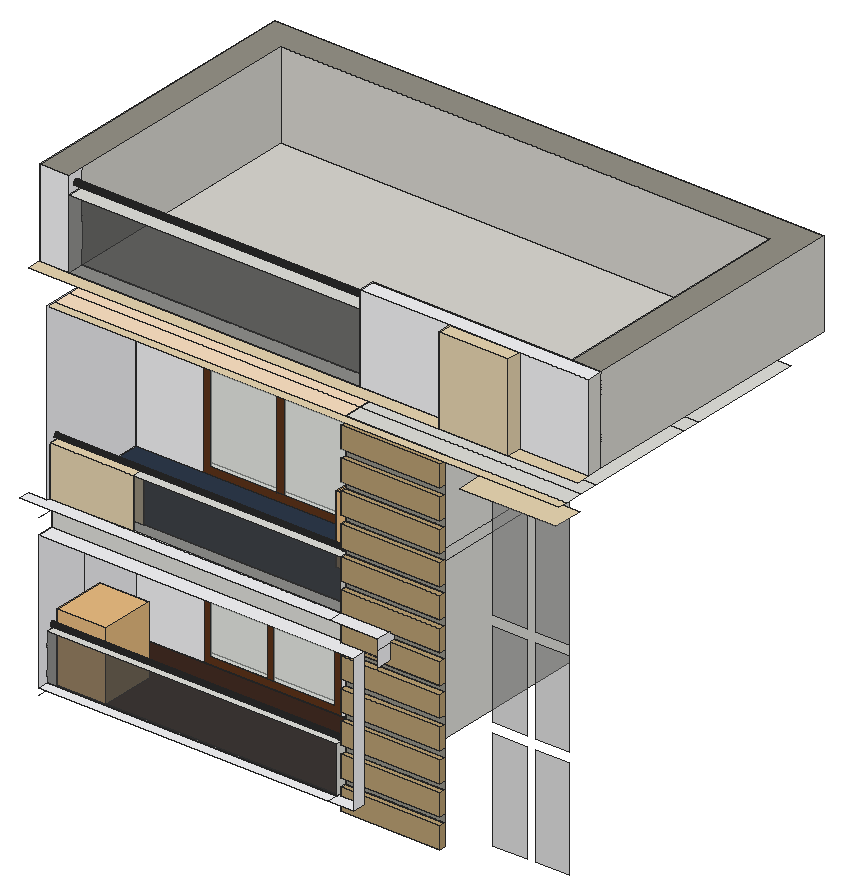
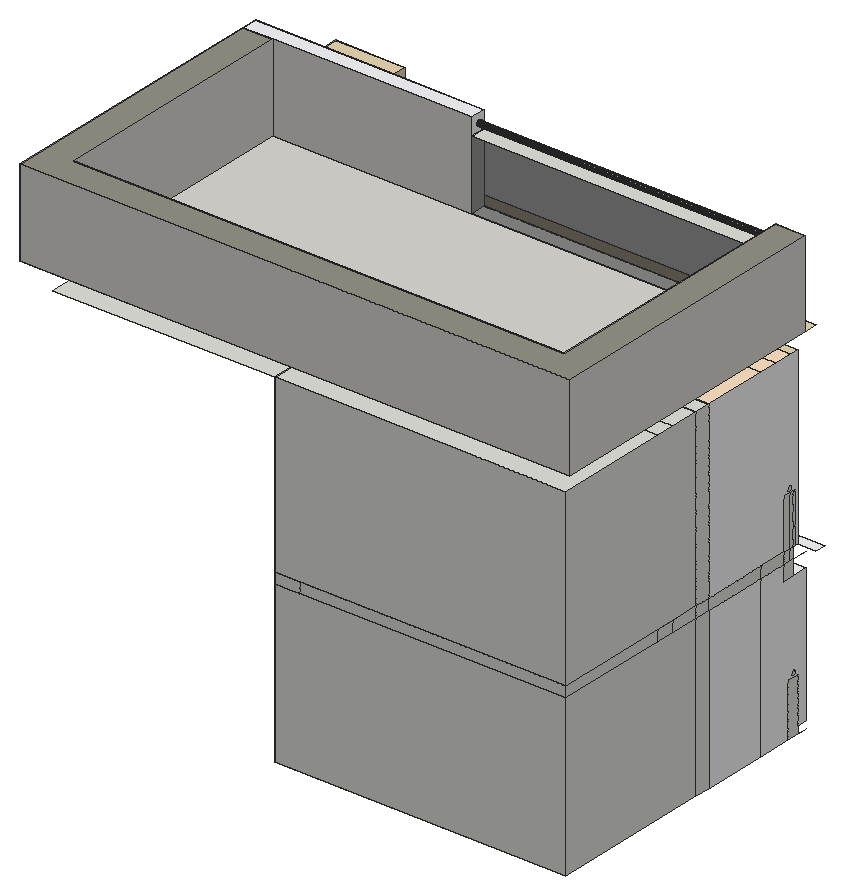
# SketchUp Ruby script. Lengths in inches.
U = 1.inch
M = Sketchup.active_model
def pt(a) = Geom::Point3d.new(a.map { |v| v * U })
def face(e, loops, mat)
  f = e.add_face(loops[0].map { |a| pt(a) })
  loops[1..].each { |l| e.add_face(l.map { |a| pt(a) }).erase! }
  f.material = f.back_material = mat if mat
  f
end
# faces: each face lists its corners as indices into pts; further lists are holes
def faces(e, pts, list, mat = nil) = list.each { |f| face(e, (f[0].is_a?(Array) ? f : [f]).map { |l| l.map { |i| pts[i] } }, mat) }
# xy, xz, yz: faces in a plane at the given z, y or x. An outline is a flat list of corners, or four numbers for a rectangle; further outlines are holes
def ring(l) = l.size == 4 ? [[l[0], l[1]], [l[2], l[1]], [l[2], l[3]], [l[0], l[3]]] : l.each_slice(2).to_a
def flat(e, list, mat, &to3) = list.each { |f| face(e, (f[0].is_a?(Array) ? f : [f]).map { |l| ring(l).map { |u, v| to3.(u, v) } }, mat) }
def xy(e, z, list, mat = nil) = flat(e, list, mat) { |x, y| [x, y, z] }
def xz(e, y, list, mat = nil) = flat(e, list, mat) { |x, z| [x, y, z] }
def yz(e, x, list, mat = nil) = flat(e, list, mat) { |y, z| [x, y, z] }
def lines(e, pts, list) = list.each { |a, b| e.add_line(pt(pts[a]), pt(pts[b])) }
# prism: a flat outline (further loops are holes) pulled along v
def prism(e, loops, v, mat = nil)
  f = face(e, loops, mat); d = Geom::Vector3d.new(v.map { |x| x * U })
  f.pushpull(f.normal.samedirection?(d) ? d.length : -d.length)
end
def box(e, o, s, mat = nil) = prism(e, [[o, [o[0] + s[0], o[1], o[2]], [o[0] + s[0], o[1] + s[1], o[2]], [o[0], o[1] + s[1], o[2]]]], [0, 0, s[2]], mat)
def at(x, y, z, deg = 0) = Geom::Transformation.translation(pt([x, y, z])) * Geom::Transformation.rotation(ORIGIN, Z_AXIS, deg.degrees)
def axes(o, x, y, z) = Geom::Transformation.new([*x, 0, *y, 0, *z, 0, *pt(o).to_a, 1])
def part(name) = M.definitions.add(name)
# library, detail: a bought-in or finely detailed component or shape, given as its bounding box
def library(name, o, s) = part(name).tap { |d| box(d.entities, o, s) }
def detail(e, o, s) = box(e.add_group.entities, o, s)
def put(e, d, t, mat = nil) = e.add_instance(d, t).tap { |i| i.material = mat if mat }
def group(e, t, mat = nil) = e.add_group.tap { |g| g.transformation = t; g.material = mat if mat }.entities
root = M.entities
M.materials.add("[0012_Bisque]").color = [255, 228, 196]
M.materials.add("[Blinds Vertical Pattern]").color = [247, 247, 249]
M.materials.add("[Formica Graystone]").color = [149, 146, 135]
M.materials.add("[Leather Blue]").color = [45, 57, 74]
M.materials.add("[Quartz Light Brown]").color = [234, 216, 179]
M.materials.add("[Suede Brown]").color = [61, 41, 32]
M.materials.add("[Terrazzo Tile Light]").color = [219, 217, 210]
M.materials.add("[Translucent Glass Gray]1").color = [68, 68, 68]
M.materials["[Translucent Glass Gray]1"].alpha = 0.5
M.materials.add("[Translucent Glass Gray]2").color = [128, 128, 128]
M.materials["[Translucent Glass Gray]2"].alpha = 0.5
M.materials.add("[Translucent Glass Safety]1").color = [237, 244, 239]
M.materials["[Translucent Glass Safety]1"].alpha = 0.5
M.materials.add("[Wood Cherry Original]").color = [94, 53, 26]
M.materials.add("[Wood Floor Light]").color = [186, 160, 115]
c1 = library("chau cay",[-24.34,-109.24,0],[56.46,62.58,79.69])
xy(root,479.875,[[484.74,326.3,600.81,332.93]],"[Wood Floor Light]")
xy(root,488.6875,[[144.51,321.91,483.06,335.74],[144.51,452.16,484.74,470.45],[144.51,470.45,484.74,660.02]])
xy(root,488.6875,[[144.51,335.74,483.06,335.74,483.06,341.61,484.74,341.61,484.74,452.16,144.51,452.16]],"[Suede Brown]")
xy(root,496.8125,[[144.51,309.6,483.06,321.91],[483.06,309.6,513.0625,309.6,513.0625,324.41,484.74,324.41,484.74,341.61,483.06,341.61]],"[Blinds Vertical Pattern]")
xy(root,504.8125,[[484.74,326.3,600.81,332.93]],"[Wood Floor Light]")
xy(root,514.3125,[[484.74,326.3,600.81,332.93]],"[Wood Floor Light]")
xy(root,539.25,[[484.74,326.3,600.81,332.93]],"[Wood Floor Light]")
xy(root,548.75,[[484.74,326.3,600.81,332.93]],"[Wood Floor Light]")
xy(root,551,[[144.51,321.91,483.06,335.74]])
xy(root,573.6875,[[484.74,326.3,600.81,332.93]],"[Wood Floor Light]")
xy(root,583.1875,[[484.74,326.3,600.81,332.93]],"[Wood Floor Light]")
xy(root,608.125,[[484.74,326.3,600.81,332.93]],"[Wood Floor Light]")
xy(root,617.625,[[484.74,326.3,600.81,332.93]],"[Wood Floor Light]")
xy(root,642.5625,[[484.74,326.3,600.81,332.93]],"[Wood Floor Light]")
xy(root,652.0625,[[484.74,326.3,600.81,332.93]],"[Wood Floor Light]")
xy(root,656.64,[[144.51,309.6,144.51,328.63,541.38,328.63,541.38,324.41,513.0625,324.41,513.0625,309.6]],"[Blinds Vertical Pattern]")
xy(root,674.6875,[[484.74,326.3,541.38,328.63],[144.51,452.16,484.74,470.45],[144.51,470.45,484.74,660.02]])
xy(root,674.6875,[[144.51,328.63,484.74,452.16]],"[0012_Bisque]")
xy(root,677,[[484.74,326.3,541.38,332.93]])
xy(root,677,[[541.38,326.3,600.81,332.93]],"[Wood Floor Light]")
xy(root,686.5,[[484.74,326.3,541.38,332.93]])
xy(root,686.5,[[541.38,326.3,600.81,332.93]],"[Wood Floor Light]")
xy(root,687.5,[[144.51,326.3,484.74,341.61],[144.51,452.16,484.74,470.45],[144.51,470.45,484.74,660.02]])
xy(root,687.5,[[123.03,309.6,484.74,309.6,484.74,326.3,144.51,326.3,144.51,321.91,123.03,321.91],[484.74,309.6,541.38,326.3]],"[Blinds Vertical Pattern]")
xy(root,687.5,[[144.51,341.61,484.74,452.16]],"[Leather Blue]")
xy(root,711.4375,[[484.74,326.3,600.81,332.93]],"[Wood Floor Light]")
xy(root,720.9375,[[484.74,326.3,600.81,332.93]],"[Wood Floor Light]")
xy(root,745.875,[[242.19,326.3,484.74,341.61]])
xy(root,745.875,[[144.51,326.3,242.19,341.61]],"[Quartz Light Brown]")
xy(root,745.875,[[484.74,326.3,600.81,332.93]],"[Wood Floor Light]")
xy(root,755.375,[[484.74,326.3,600.81,332.93]],"[Wood Floor Light]")
xy(root,780.3125,[[484.74,326.3,600.81,332.93]],"[Wood Floor Light]")
xy(root,789.8125,[[484.74,326.3,600.81,332.93]],"[Wood Floor Light]")
xy(root,814.75,[[484.74,326.3,600.81,332.93]],"[Wood Floor Light]")
xy(root,824.25,[[484.74,326.3,600.81,332.93]],"[Wood Floor Light]")
xy(root,849.1875,[[484.74,326.3,600.81,332.93]],"[Wood Floor Light]")
xy(root,858.6875,[[484.74,326.3,600.81,332.93]],"[Wood Floor Light]")
xy(root,861.54,[[618.4,332.93,730.9,367.24]],"[Quartz Light Brown]")
xy(root,883.625,[[484.74,326.3,600.81,332.93]],"[Wood Floor Light]")
xy(root,890.6875,[[484.74,332.93,743.35,353.85],[484.74,353.85,743.35,375.33],[484.74,375.33,743.35,504.41],[144.51,452.16,484.74,470.45],[144.51,470.45,484.74,504.41],
  [144.51,504.41,484.74,525.85],[484.74,504.41,743.35,525.85],[144.51,525.85,484.74,660.02],[484.74,525.85,743.35,660.02]])
xy(root,890.6875,[[144.51,332.93,484.74,353.85],[144.51,353.85,484.74,375.33],[144.51,375.33,484.74,452.16]],"[0012_Bisque]")
xy(root,890.6875,[[144.51,321.91,743.35,332.93]],"[Quartz Light Brown]")
xy(root,923.6875,[[603.0625,321.91,683.95,338.07],[123.03,338.07,123.03,681.5,764.83,681.5,764.83,356.55,730.2,356.55,730.2,646.87,157.66,646.87,157.66,338.07],[157.66,338.07,497.79,356.55],[497.79,338.07,764.83,356.55]])
xy(root,923.6875,[[123.03,321.91,603.0625,338.07],[683.95,321.91,764.83,338.07]],"[Quartz Light Brown]")
xy(root,923.6875,[[157.66,356.55,730.2,646.87]],"[Terrazzo Tile Light]")
xy(root,1005.0625,[[157.66,338.07,497.79,356.55]])
xy(root,1024.8125,[[497.79,338.07,764.83,356.55]],"[Blinds Vertical Pattern]")
xy(root,1024.8125,[[123.03,338.07,157.66,338.07,157.66,646.87,730.2,646.87,730.2,356.55,764.83,356.55,764.83,681.5,123.03,681.5]],"[Formica Graystone]")
xy(root,1024.8125,[[603.0625,321.91,683.95,338.07]],"[Quartz Light Brown]")
xz(root,321.91,[[144.51,488.6875,483.06,496.8125]])
xz(root,321.91,[[603.0625,923.6875,683.95,1024.8125]],"[Quartz Light Brown]")
xz(root,321.91,[[144.51,496.8125,483.06,551]],"[Translucent Glass Gray]1")
xz(root,326.3,[[484.74,674.6875,541.38,677],[484.74,686.5,541.38,687.5]])
xz(root,326.3,[[144.51,687.5,242.19,745.875]],"[Quartz Light Brown]")
xz(root,326.3,[[242.19,687.5,484.74,745.875]],"[Translucent Glass Gray]1")
xz(root,326.3,[[484.74,479.875,600.81,504.8125],[484.74,514.3125,600.81,539.25],[484.74,548.75,600.81,573.6875],[484.74,583.1875,600.81,608.125],[484.74,617.625,600.81,642.5625],
  [484.74,652.0625,600.81,652.0625,600.81,677,541.38,677,541.38,674.6875,484.74,674.6875],[541.38,686.5,600.81,686.5,600.81,711.4375,484.74,711.4375,484.74,687.5,541.38,687.5],[484.74,720.9375,600.81,745.875],[484.74,755.375,600.81,780.3125],[484.74,789.8125,600.81,814.75],
  [484.74,824.25,600.81,849.1875],[484.74,858.6875,600.81,883.625]],"[Wood Floor Light]")
xz(root,328.63,[[144.51,656.64,541.38,674.6875]])
xz(root,332.93,[[484.74,479.875,600.81,504.8125],[484.74,514.3125,600.81,539.25],[484.74,548.75,600.81,573.6875],[484.74,583.1875,600.81,608.125],[484.74,617.625,600.81,642.5625],
  [484.74,652.0625,600.81,677],[484.74,677,541.38,686.5],[484.74,686.5,600.81,711.4375],[484.74,720.9375,600.81,745.875],[484.74,755.375,600.81,780.3125],
  [484.74,789.8125,600.81,814.75],[484.74,824.25,600.81,849.1875],[484.74,858.6875,600.81,883.625]])
xz(root,332.93,[[484.74,504.8125,600.81,514.3125],[484.74,539.25,600.81,548.75],[484.74,573.6875,600.81,583.1875],[484.74,608.125,600.81,617.625],[484.74,642.5625,600.81,652.0625],
  [541.38,677,600.81,686.5],[484.74,711.4375,600.81,720.9375],[484.74,745.875,600.81,755.375],[484.74,780.3125,600.81,789.8125],[484.74,814.75,600.81,824.25],
  [484.74,849.1875,600.81,858.6875],[484.74,883.625,600.81,890.6875]],"[Formica Graystone]")
xz(root,335.74,[[144.51,488.6875,483.06,551]],"[Translucent Glass Gray]1")
xz(root,338.07,[[603.0625,923.6875,683.95,1024.8125]])
xz(root,338.07,[[123.03,923.6875,157.66,1024.8125],[497.79,923.6875,603.0625,1024.8125],[683.95,923.6875,764.83,1024.8125]],"[Blinds Vertical Pattern]")
xz(root,338.07,[[157.66,923.6875,497.79,1005.0625]],"[Translucent Glass Gray]1")
xz(root,341.61,[[483.06,488.6875,484.74,496.8125]])
xz(root,341.61,[[144.51,687.5,242.19,745.875]],"[Quartz Light Brown]")
xz(root,341.61,[[242.19,687.5,484.74,745.875]],"[Translucent Glass Gray]1")
xz(root,356.55,[[730.2,923.6875,764.83,1024.8125]])
xz(root,356.55,[[497.79,923.6875,730.2,1024.8125]],"[Terrazzo Tile Light]")
xz(root,356.55,[[157.66,923.6875,497.79,1005.0625]],"[Translucent Glass Gray]1")
xz(root,367.24,[[630.125,475.62,670.08,594.34],[679.79,475.62,719.18,594.34],[630.125,604.84,670.08,706.4],[679.79,604.84,719.18,706.4],[630.125,716.91,670.08,849.82],
  [679.79,716.91,719.18,849.82]],"[Translucent Glass Gray]2")
xz(root,452.16,[[144.51,488.6875,223.62,488.6875,223.62,650.375,385.3,650.375,385.3,488.6875,484.74,488.6875,484.74,674.6875,144.51,674.6875],[144.51,687.5,222.91,687.5,222.91,869.9375,405.34,869.9375,405.34,687.5,484.74,687.5,484.74,890.6875,144.51,890.6875]],"[Blinds Vertical Pattern]")
xz(root,452.16,[[231.79,496.86,298.09,642.2],[305.3125,496.86,377.13,642.2],[231.78,696.375,308.83,861.0625],[318.94,696.375,396.47,861.0625]],"[Translucent Glass Safety]1")
xz(root,452.16,[[[223.62,488.6875,385.3,650.375],[231.79,496.86,377.13,642.2]],[298.09,496.86,305.3125,642.2],[[222.91,687.5,405.34,869.9375],[231.78,696.375,396.47,861.0625]],[308.83,696.375,318.94,861.0625]],"[Wood Cherry Original]")
xz(root,470.45,[[144.51,488.6875,484.74,674.6875],[144.51,687.5,484.74,890.6875]])
xz(root,646.87,[[157.66,923.6875,730.2,1024.8125]],"[Terrazzo Tile Light]")
xz(root,660.02,[[144.51,488.6875,484.74,674.6875],[144.51,674.6875,455.26,687.5],[455.26,674.6875,484.74,687.5],[144.51,687.5,484.74,890.6875]])
xz(root,681.5,[[123.03,923.6875,764.83,1024.8125]],"[Terrazzo Tile Light]")
yz(root,123.03,[[338.07,923.6875,681.5,1024.8125]],"[Terrazzo Tile Light]")
yz(root,144.51,[[321.91,488.6875,335.74,551],[452.16,488.6875,470.45,674.6875],[470.45,488.6875,660.02,674.6875],[328.4,553.4,327.82,553.48,327.28,553.71,326.8125,554.0625,326.45,554.53,326.23,555.07,326.15,555.65,326.23,556.24,326.45,556.78,326.8125,557.24,327.28,557.6,327.82,557.83,328.4,557.9,328.98,557.83,329.53,557.6,329.99,557.24,330.35,556.78,330.58,556.24,330.65,555.65,330.58,555.07,330.35,554.53,329.99,554.0625,329.53,553.71,328.98,553.48],[328.63,656.64,341.61,674.6875],
  [328.63,674.6875,332.93,687.5],[332.93,674.6875,341.61,687.5],[341.61,674.6875,375.33,687.5],[375.33,674.6875,452.16,687.5],[452.16,674.6875,470.45,687.5],
  [470.45,674.6875,504.41,687.5],[504.41,674.6875,525.85,687.5],[525.85,674.6875,660.02,687.5],[326.3,687.5,328.63,745.875],[328.63,687.5,332.93,745.875],
  [332.93,687.5,341.61,745.875],[452.16,687.5,470.45,890.6875],[470.45,687.5,660.02,890.6875],[334.17,748.4,333.54,748.49,332.95,748.73,332.44,749.12,332.06,749.62,331.8125,750.21,331.73,750.84,331.8125,751.47,332.06,752.06,332.44,752.5625,332.95,752.95,333.54,753.19,334.17,753.28,334.8,753.19,335.39,752.95,335.89,752.5625,336.28,752.06,336.52,751.47,336.6,750.84,336.52,750.21,336.28,749.62,335.89,749.12,335.39,748.73,334.8,748.49]])
yz(root,144.51,[[[335.74,488.6875,375.33,488.6875,375.33,674.6875,341.61,674.6875,341.61,656.64,309.6,656.64,309.6,496.8125,321.91,496.8125,321.91,551,335.74,551],[328.4,553.4,327.82,553.48,327.28,553.71,326.8125,554.0625,326.45,554.53,326.23,555.07,326.15,555.65,326.23,556.24,326.45,556.78,326.8125,557.24,327.28,557.6,327.82,557.83,328.4,557.9,328.98,557.83,329.53,557.6,329.99,557.24,330.35,556.78,330.58,556.24,330.65,555.65,330.58,555.07,330.35,554.53,329.99,554.0625,329.53,553.71,328.98,553.48]],[375.33,488.6875,452.16,674.6875],[[321.91,687.5,326.3,687.5,326.3,745.875,341.61,745.875,341.61,687.5,452.16,687.5,452.16,890.6875,321.91,890.6875],[334.17,748.4,333.54,748.49,332.95,748.73,332.44,749.12,332.06,749.62,331.8125,750.21,331.73,750.84,331.8125,751.47,332.06,752.06,332.44,752.5625,332.95,752.95,333.54,753.19,334.17,753.28,334.8,753.19,335.39,752.95,335.89,752.5625,336.28,752.06,336.52,751.47,336.6,750.84,336.52,750.21,336.28,749.62,335.89,749.12,335.39,748.73,334.8,748.49]]],"[Blinds Vertical Pattern]")
yz(root,157.66,[[338.07,923.6875,356.55,1005.0625],[346.8125,1012.1,346.07,1012.19,345.375,1012.48,344.78,1012.9375,344.32,1013.53,344.03,1014.23,343.9375,1014.97,344.03,1015.72,344.32,1016.41,344.78,1017,345.375,1017.46,346.07,1017.75,346.8125,1017.85,347.56,1017.75,348.25,1017.46,348.84,1017,349.3,1016.41,349.59,1015.72,349.6875,1014.97,349.59,1014.23,349.3,1013.53,348.84,1012.9375,348.25,1012.48,347.56,1012.19]])
yz(root,157.66,[[[338.07,1005.0625,356.55,1024.8125],[346.8125,1012.1,346.07,1012.19,345.375,1012.48,344.78,1012.9375,344.32,1013.53,344.03,1014.23,343.9375,1014.97,344.03,1015.72,344.32,1016.41,344.78,1017,345.375,1017.46,346.07,1017.75,346.8125,1017.85,347.56,1017.75,348.25,1017.46,348.84,1017,349.3,1016.41,349.59,1015.72,349.6875,1014.97,349.59,1014.23,349.3,1013.53,348.84,1012.9375,348.25,1012.48,347.56,1012.19]]],"[Blinds Vertical Pattern]")
yz(root,157.66,[[356.55,923.6875,646.87,1024.8125]],"[Terrazzo Tile Light]")
yz(root,483.06,[[321.91,488.6875,335.74,496.8125],[335.74,488.6875,341.61,496.8125],[321.91,496.8125,335.74,551]])
yz(root,484.74,[[326.3,479.875,332.93,496.8125],[452.16,488.6875,470.45,674.6875],[470.45,488.6875,660.02,674.6875],[326.3,496.8125,332.93,504.8125],[326.3,514.3125,332.93,539.25],
  [328.4,553.4,327.82,553.48,327.28,553.71,326.8125,554.0625,326.45,554.53,326.3,554.9,326.3,556.41,326.45,556.78,326.8125,557.24,327.28,557.6,327.82,557.83,328.4,557.9,328.98,557.83,329.53,557.6,329.99,557.24,330.35,556.78,330.58,556.24,330.65,555.65,330.58,555.07,330.35,554.53,329.99,554.0625,329.53,553.71,328.98,553.48],[326.3,554.9,326.3,556.41,326.23,556.24,326.15,555.65,326.23,555.07],[326.3,674.6875,332.93,677],[332.93,674.6875,660.02,687.5],[326.3,686.5,332.93,687.5],
  [326.3,687.5,332.93,711.4375],[332.93,687.5,341.61,745.875],[452.16,687.5,470.45,890.6875],[470.45,687.5,660.02,890.6875],[326.3,711.4375,332.93,720.9375],
  [326.3,720.9375,332.93,745.875],[334.17,748.4,333.54,748.49,332.95,748.73,332.93,748.75,332.93,752.93,332.95,752.95,333.54,753.19,334.17,753.28,334.8,753.19,335.39,752.95,335.89,752.5625,336.28,752.06,336.52,751.47,336.6,750.84,336.52,750.21,336.28,749.62,335.89,749.12,335.39,748.73,334.8,748.49],[332.93,748.75,332.93,752.93,332.44,752.5625,332.06,752.06,331.8125,751.47,331.73,750.84,331.8125,750.21,332.06,749.62,332.44,749.12]])
yz(root,484.74,[[341.61,488.6875,341.61,496.8125,332.93,496.8125,332.93,674.6875,452.16,674.6875,452.16,488.6875],[341.61,687.5,341.61,745.875,332.93,745.875,332.93,748.75,332.95,748.73,333.54,748.49,334.17,748.4,334.8,748.49,335.39,748.73,335.89,749.12,336.28,749.62,336.52,750.21,336.6,750.84,336.52,751.47,336.28,752.06,335.89,752.5625,335.39,752.95,334.8,753.19,334.17,753.28,333.54,753.19,332.95,752.95,332.93,752.93,332.93,890.6875,452.16,890.6875,452.16,687.5]],"[Blinds Vertical Pattern]")
yz(root,484.74,[[326.3,548.75,326.3,554.9,326.45,554.53,326.8125,554.0625,327.28,553.71,327.82,553.48,328.4,553.4,328.98,553.48,329.53,553.71,329.99,554.0625,330.35,554.53,330.58,555.07,330.65,555.65,330.58,556.24,330.35,556.78,329.99,557.24,329.53,557.6,328.98,557.83,328.4,557.9,327.82,557.83,327.28,557.6,326.8125,557.24,326.45,556.78,326.3,556.41,326.3,573.6875,332.93,573.6875,332.93,548.75],[326.3,583.1875,332.93,608.125],[326.3,617.625,332.93,642.5625],[326.3,652.0625,332.93,674.6875],[326.3,755.375,332.93,780.3125],
  [326.3,789.8125,332.93,814.75],[326.3,824.25,332.93,849.1875],[326.3,858.6875,332.93,883.625]],"[Wood Floor Light]")
yz(root,497.79,[[338.07,923.6875,356.55,1005.0625]])
yz(root,497.79,[[[338.07,1005.0625,356.55,1024.8125],[346.8125,1012.1,347.56,1012.19,348.25,1012.48,348.84,1012.9375,349.3,1013.53,349.59,1014.23,349.6875,1014.97,349.59,1015.72,349.3,1016.41,348.84,1017,348.25,1017.46,347.56,1017.75,346.8125,1017.85,346.07,1017.75,345.375,1017.46,344.78,1017,344.32,1016.41,344.03,1015.72,343.9375,1014.97,344.03,1014.23,344.32,1013.53,344.78,1012.9375,345.375,1012.48,346.07,1012.19]]],"[Blinds Vertical Pattern]")
yz(root,513.0625,[[309.6,496.8125,324.41,656.64]],"[Blinds Vertical Pattern]")
yz(root,541.38,[[309.6,656.64,328.63,674.6875],[309.6,674.6875,326.3,674.6875,326.3,677,332.93,677,332.93,686.5,326.3,686.5,326.3,687.5,309.6,687.5]],"[Blinds Vertical Pattern]")
yz(root,600.81,[[326.3,479.875,332.93,504.8125],[326.3,514.3125,332.93,539.25],[326.3,548.75,332.93,573.6875],[326.3,583.1875,332.93,608.125],[326.3,617.625,332.93,642.5625],
  [326.3,652.0625,332.93,677],[326.3,686.5,332.93,711.4375],[326.3,720.9375,332.93,745.875],[326.3,755.375,332.93,780.3125],[326.3,789.8125,332.93,814.75],
  [326.3,824.25,332.93,849.1875],[326.3,858.6875,332.93,883.625]],"[Wood Floor Light]")
yz(root,603.0625,[[321.91,923.6875,338.07,1024.8125]],"[Quartz Light Brown]")
yz(root,683.95,[[321.91,923.6875,338.07,1024.8125]],"[Quartz Light Brown]")
yz(root,730.2,[[356.55,923.6875,646.87,1024.8125]],"[Terrazzo Tile Light]")
yz(root,764.83,[[338.07,923.6875,356.55,1024.8125],[356.55,923.6875,681.5,1024.8125]],"[Terrazzo Tile Light]")
p = [[144.51,327.82,553.48],[144.51,328.4,553.4],[484.74,328.4,553.4],[484.74,327.82,553.48],[144.51,328.98,553.48],[484.74,328.98,553.48],
  [144.51,327.28,553.71],[484.74,327.28,553.71],[144.51,329.53,553.71],[484.74,329.53,553.71],[144.51,326.8125,554.0625],[484.74,326.8125,554.0625],
  [144.51,329.99,554.0625],[484.74,329.99,554.0625],[144.51,326.45,554.53],[484.74,326.45,554.53],[144.51,330.35,554.53],[484.74,330.35,554.53],
  [144.51,326.23,555.07],[484.74,326.3,554.9],[484.74,326.23,555.07],[144.51,330.58,555.07],[484.74,330.58,555.07],[144.51,326.15,555.65],
  [484.74,326.15,555.65],[144.51,330.65,555.65],[484.74,330.65,555.65],[144.51,326.23,556.24],[484.74,326.23,556.24],[144.51,330.58,556.24],
  [484.74,330.58,556.24],[144.51,326.45,556.78],[484.74,326.3,556.41],[484.74,326.45,556.78],[144.51,330.35,556.78],[484.74,330.35,556.78],
  [144.51,326.8125,557.24],[484.74,326.8125,557.24],[144.51,329.99,557.24],[484.74,329.99,557.24],[144.51,327.28,557.6],[484.74,327.28,557.6],
  [144.51,329.53,557.6],[484.74,329.53,557.6],[144.51,327.82,557.83],[484.74,327.82,557.83],[144.51,328.98,557.83],[484.74,328.98,557.83],
  [144.51,328.4,557.9],[484.74,328.4,557.9],[144.51,333.54,748.49],[144.51,334.17,748.4],[484.74,334.17,748.4],[484.74,333.54,748.49],
  [144.51,334.8,748.49],[484.74,334.8,748.49],[144.51,332.95,748.73],[484.74,332.95,748.73],[144.51,335.39,748.73],[484.74,335.39,748.73],
  [144.51,332.44,749.12],[484.74,332.93,748.75],[484.74,332.44,749.12],[144.51,335.89,749.12],[484.74,335.89,749.12],[144.51,332.06,749.62],
  [484.74,332.06,749.62],[144.51,336.28,749.62],[484.74,336.28,749.62],[144.51,331.8125,750.21],[484.74,331.8125,750.21],[144.51,336.52,750.21],
  [484.74,336.52,750.21],[144.51,331.73,750.84],[484.74,331.73,750.84],[144.51,336.6,750.84],[484.74,336.6,750.84],[144.51,331.8125,751.47],
  [484.74,331.8125,751.47],[144.51,336.52,751.47],[484.74,336.52,751.47],[144.51,332.06,752.06],[484.74,332.06,752.06],[144.51,336.28,752.06],
  [484.74,336.28,752.06],[144.51,332.44,752.5625],[484.74,332.44,752.5625],[144.51,335.89,752.5625],[484.74,335.89,752.5625],[144.51,332.95,752.95],
  [484.74,332.93,752.93],[484.74,332.95,752.95],[144.51,335.39,752.95],[484.74,335.39,752.95],[144.51,333.54,753.19],[484.74,333.54,753.19],
  [144.51,334.8,753.19],[484.74,334.8,753.19],[144.51,334.17,753.28],[484.74,334.17,753.28],[157.66,346.07,1012.19],[157.66,346.8125,1012.1],
  [497.79,346.8125,1012.1],[497.79,346.07,1012.19],[157.66,347.56,1012.19],[497.79,347.56,1012.19],[157.66,345.375,1012.48],[497.79,345.375,1012.48],
  [157.66,348.25,1012.48],[497.79,348.25,1012.48],[157.66,344.78,1012.9375],[497.79,344.78,1012.9375],[157.66,348.84,1012.9375],[497.79,348.84,1012.9375],
  [157.66,344.32,1013.53],[497.79,344.32,1013.53],[157.66,349.3,1013.53],[497.79,349.3,1013.53],[157.66,344.03,1014.23],[497.79,344.03,1014.23],
  [157.66,349.59,1014.23],[497.79,349.59,1014.23],[157.66,343.9375,1014.97],[497.79,343.9375,1014.97],[157.66,349.6875,1014.97],[497.79,349.6875,1014.97],
  [157.66,344.03,1015.72],[497.79,344.03,1015.72],[157.66,349.59,1015.72],[497.79,349.59,1015.72],[157.66,344.32,1016.41],[497.79,344.32,1016.41],
  [157.66,349.3,1016.41],[497.79,349.3,1016.41],[157.66,344.78,1017],[497.79,344.78,1017],[157.66,348.84,1017],[497.79,348.84,1017],
  [157.66,345.375,1017.46],[497.79,345.375,1017.46],[157.66,348.25,1017.46],[497.79,348.25,1017.46],[157.66,346.07,1017.75],[497.79,346.07,1017.75],
  [157.66,347.56,1017.75],[497.79,347.56,1017.75],[157.66,346.8125,1017.85],[497.79,346.8125,1017.85],[144.51,321.91,488.6875],[144.51,309.6,488.6875],
  [144.51,328.63,674.6875],[144.51,309.6,674.6875]]
faces(root,p,[[0,1,2,3],[1,4,5,2],[6,0,3,7],[4,8,9,5],[10,6,7,11],[8,12,13,9],[14,10,11,15],[12,16,17,13],
  [18,14,15,19,20],[16,21,22,17],[23,18,20,24],[21,25,26,22],[27,23,24,28],[25,29,30,26],[31,27,28,32,33],[29,34,35,30],
  [36,31,33,37],[34,38,39,35],[40,36,37,41],[38,42,43,39],[44,40,41,45],[42,46,47,43],[48,44,45,49],[46,48,49,47],
  [50,51,52,53],[51,54,55,52],[56,50,53,57],[54,58,59,55],[60,56,57,61,62],[58,63,64,59],[65,60,62,66],[63,67,68,64],
  [69,65,66,70],[67,71,72,68],[73,69,70,74],[71,75,76,72],[77,73,74,78],[75,79,80,76],[81,77,78,82],[79,83,84,80],
  [85,81,82,86],[83,87,88,84],[89,85,86,90,91],[87,92,93,88],[94,89,91,95],[92,96,97,93],[98,94,95,99],[96,98,99,97],
  [100,101,102,103],[101,104,105,102],[106,100,103,107],[104,108,109,105],[110,106,107,111],[108,112,113,109],[114,110,111,115],[112,116,117,113],
  [118,114,115,119],[116,120,121,117],[122,118,119,123],[120,124,125,121],[126,122,123,127],[124,128,129,125],[130,126,127,131],[128,132,133,129],
  [134,130,131,135],[132,136,137,133],[138,134,135,139],[136,140,141,137],[142,138,139,143],[140,144,145,141],[146,142,143,147],[144,146,147,145]],"[Quartz Light Brown]")
lines(root,p,[[148,149],[150,151]])
put(root,c1,at(170.21,444.64,488.6875))
put(root,c1,at(452.62,498.82,687.5))
